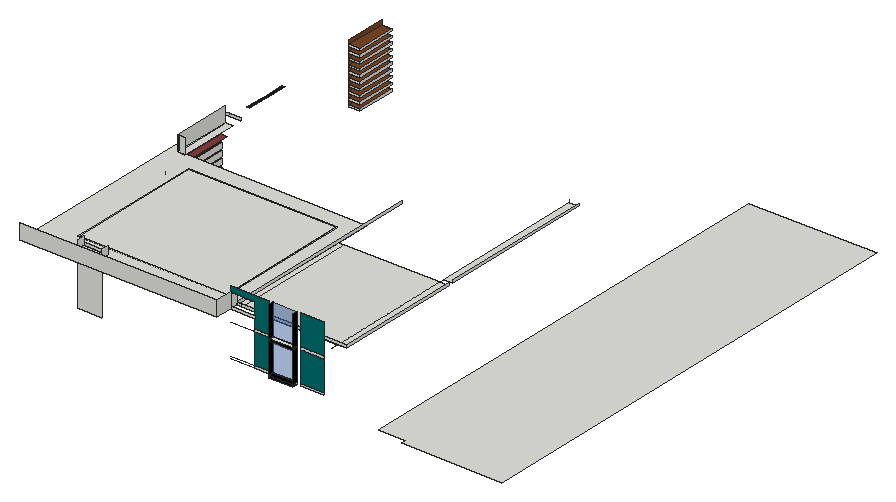
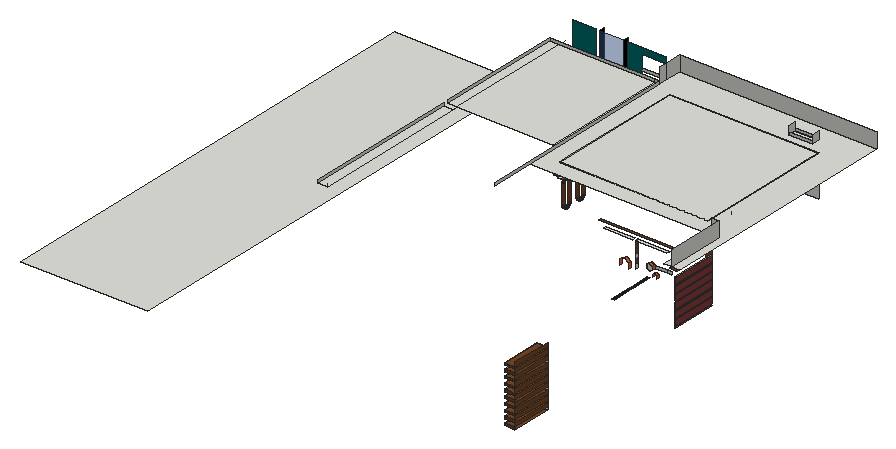
# SketchUp Ruby script. Lengths in inches.
U = 1.inch
M = Sketchup.active_model
def pt(a) = Geom::Point3d.new(a.map { |v| v * U })
def face(e, loops, mat)
  f = e.add_face(loops[0].map { |a| pt(a) })
  loops[1..].each { |l| e.add_face(l.map { |a| pt(a) }).erase! }
  f.material = f.back_material = mat if mat
  f
end
# faces: each face lists its corners as indices into pts; further lists are holes
def faces(e, pts, list, mat = nil) = list.each { |f| face(e, (f[0].is_a?(Array) ? f : [f]).map { |l| l.map { |i| pts[i] } }, mat) }
# xy, xz, yz: faces in a plane at the given z, y or x. An outline is a flat list of corners, or four numbers for a rectangle; further outlines are holes
def ring(l) = l.size == 4 ? [[l[0], l[1]], [l[2], l[1]], [l[2], l[3]], [l[0], l[3]]] : l.each_slice(2).to_a
def flat(e, list, mat, &to3) = list.each { |f| face(e, (f[0].is_a?(Array) ? f : [f]).map { |l| ring(l).map { |u, v| to3.(u, v) } }, mat) }
def xy(e, z, list, mat = nil) = flat(e, list, mat) { |x, y| [x, y, z] }
def xz(e, y, list, mat = nil) = flat(e, list, mat) { |x, z| [x, y, z] }
def yz(e, x, list, mat = nil) = flat(e, list, mat) { |y, z| [x, y, z] }
def lines(e, pts, list) = list.each { |a, b| e.add_line(pt(pts[a]), pt(pts[b])) }
# prism: a flat outline (further loops are holes) pulled along v
def prism(e, loops, v, mat = nil)
  f = face(e, loops, mat); d = Geom::Vector3d.new(v.map { |x| x * U })
  f.pushpull(f.normal.samedirection?(d) ? d.length : -d.length)
end
def box(e, o, s, mat = nil) = prism(e, [[o, [o[0] + s[0], o[1], o[2]], [o[0] + s[0], o[1] + s[1], o[2]], [o[0], o[1] + s[1], o[2]]]], [0, 0, s[2]], mat)
def at(x, y, z, deg = 0) = Geom::Transformation.translation(pt([x, y, z])) * Geom::Transformation.rotation(ORIGIN, Z_AXIS, deg.degrees)
def axes(o, x, y, z) = Geom::Transformation.new([*x, 0, *y, 0, *z, 0, *pt(o).to_a, 1])
def part(name) = M.definitions.add(name)
# library, detail: a bought-in or finely detailed component or shape, given as its bounding box
def library(name, o, s) = part(name).tap { |d| box(d.entities, o, s) }
def detail(e, o, s) = box(e.add_group.entities, o, s)
def put(e, d, t, mat = nil) = e.add_instance(d, t).tap { |i| i.material = mat if mat }
def group(e, t, mat = nil) = e.add_group.tap { |g| g.transformation = t; g.material = mat if mat }.entities
root = M.entities
M.materials.add("[0017_IndianRed]").color = [135, 60, 60]
M.materials.add("[Color A08]").color = [102, 0, 0]
M.materials.add("[Color B04]").color = [255, 101, 50]
M.materials.add("[Color C07]").color = [153, 76, 0]
M.materials.add("[Color H07]1").color = [0, 109, 109]
M.materials.add("[Color M08]").color = [30, 30, 30]
M.materials.add("[Color M09]").color = [0, 0, 0]
M.materials.add("[Translucent Glass Blue]1").color = [78, 117, 186]
M.materials["[Translucent Glass Blue]1"].alpha = 0.5
M.materials.add("[Wood Veneer 01]").color = [120, 70, 37]
xy(root,186.12,[[82.23,313.6,84.23,364.52]],"[0017_IndianRed]")
xy(root,187.92,[[77.54,552.74,89.54,598.37]],"[Wood Veneer 01]")
xy(root,188.35,[[82.23,313.6,84.23,364.52]],"[0017_IndianRed]")
xy(root,188.93,[[493.41,106.91,607.41,106.91,607.41,636.48,463.41,636.48,463.41,112.91,493.41,112.91]])
xy(root,190.33,[[77.54,552.74,89.54,598.37]],"[Wood Veneer 01]")
xy(root,194.62,[[82.23,313.6,84.23,364.52]],"[0017_IndianRed]")
xy(root,194.74,[[77.54,552.74,89.54,598.37]],"[Wood Veneer 01]")
xy(root,196.85,[[82.23,313.6,84.23,364.52]],"[0017_IndianRed]")
xy(root,197.14,[[77.54,552.74,89.54,598.37]],"[Wood Veneer 01]")
xy(root,201.55,[[77.54,552.74,89.54,598.37]],"[Wood Veneer 01]")
xy(root,202.34,[[343.08,106.91,369.95,112.91]],"[Color M09]")
xy(root,203.12,[[82.23,313.6,84.23,364.52]],"[0017_IndianRed]")
xy(root,203.95,[[77.54,552.74,89.54,598.37]],"[Wood Veneer 01]")
xy(root,204.72,[[343.08,106.91,369.95,112.91]],"[Color M09]")
xy(root,205.35,[[82.23,313.6,84.23,364.52]],"[0017_IndianRed]")
xy(root,208.36,[[77.54,552.74,89.54,598.37]],"[Wood Veneer 01]")
xy(root,210.77,[[77.54,552.74,89.54,598.37]],"[Wood Veneer 01]")
xy(root,211.62,[[82.23,313.6,84.23,364.52]],"[0017_IndianRed]")
xy(root,213.85,[[82.23,313.6,84.23,364.52]],"[0017_IndianRed]")
xy(root,215.17,[[77.54,552.74,89.54,598.37]],"[Wood Veneer 01]")
xy(root,216.61,[[139.47,302.6,175.47,305.6],[178.47,302.6,211.47,305.6]])
xy(root,217.58,[[77.54,552.74,89.54,598.37]],"[Wood Veneer 01]")
xy(root,220.12,[[82.23,313.6,84.23,364.52]],"[0017_IndianRed]")
xy(root,220.55,[[291.79,229.6,291.79,243.65,288.79,243.65,288.79,247.85,291.79,247.85,291.79,266.1,294.79,266.1,294.79,229.6]])
xy(root,220.55,[[288.79,229.6,291.79,243.65],[288.79,247.85,291.79,266.1]],"[Wood Veneer 01]")
xy(root,221.99,[[77.54,552.74,89.54,598.37]],"[Wood Veneer 01]")
xy(root,222.35,[[82.23,313.6,84.23,364.52]],"[0017_IndianRed]")
xy(root,222.61,[[133.47,302.6,217.47,305.6]],"[Wood Veneer 01]")
xy(root,224.39,[[77.54,552.74,89.54,598.37]],"[Wood Veneer 01]")
xy(root,224.91,[[291.79,170.29,294.79,183.63],[291.79,186.63,294.79,202.98]])
xy(root,226.55,[[288.79,223.6,294.79,272.1]],"[Wood Veneer 01]")
xy(root,227.91,[[291.79,167.29,294.79,205.98]],"[Color M08]")
xy(root,228.62,[[82.23,313.6,84.23,364.52]],"[0017_IndianRed]")
xy(root,228.8,[[77.54,552.74,89.54,598.37]],"[Wood Veneer 01]")
xy(root,230.85,[[82.23,313.6,84.23,364.52]],"[0017_IndianRed]")
xy(root,231.2,[[77.54,552.74,89.54,598.37]],"[Wood Veneer 01]")
xy(root,235.61,[[77.54,552.74,89.54,598.37]],"[Wood Veneer 01]")
xy(root,237.12,[[82.23,313.6,84.23,364.52]],"[0017_IndianRed]")
xy(root,238.02,[[77.54,552.74,89.54,598.37]],"[Wood Veneer 01]")
xy(root,239.34,[[343.08,106.91,369.95,112.91]],"[Color M09]")
xy(root,241.72,[[343.08,106.91,369.95,112.91]])
xy(root,242.42,[[77.54,552.74,89.54,598.37]],"[Wood Veneer 01]")
xy(root,244.62,[[80.6,313.6,82.23,364.52],[82.23,313.6,89.54,364.52]],"[0017_IndianRed]")
xy(root,244.83,[[77.54,552.74,89.54,598.37]],"[Wood Veneer 01]")
xy(root,246.61,[[[115.8,139.1875,115.8125,140.26,115.8125,279.33,268.52,279.33,268.52,139.1875],[124.47,144.14,143.78,269.32],[151.22,144.14,170.53,269.32],[177.97,144.14,197.28,269.32],[204.72,144.14,224.03,269.32],[231.47,144.14,250.78,269.32]]],"[Color A08]")
xy(root,249.24,[[77.54,552.74,89.54,598.37]],"[Wood Veneer 01]")
xy(root,249.61,[[124.47,144.14,143.78,269.32],[151.22,144.14,170.53,269.32],[177.97,144.14,197.28,269.32],[204.72,144.14,224.03,269.32],[231.47,144.14,250.78,269.32]])
xy(root,249.61,[[[107.85,131.3,107.92,140.3,107.92,287.22,276.41,287.22,276.41,131.3],[115.8,139.1875,268.52,139.1875,268.52,279.33,115.8125,279.33,115.8125,140.26]]],"[Color A08]")
xy(root,251.64,[[77.54,552.74,89.54,598.37]],"[Wood Veneer 01]")
xy(root,252.61,[[[72.04,94.04,72.04,372.52,80.6,372.52,80.6,305.6,294.79,305.6,294.79,94.04],[107.85,131.3,276.41,131.3,276.41,287.22,107.92,287.22,107.92,140.3],[121.875,112.91,149.09,121.91]],[121.875,112.91,149.09,121.91],[294.79,121.91,300.66,266.1],[300.66,121.91,300.79,266.1],[300.79,121.91,409.01,266.1],
  [409.01,121.91,419.79,266.1],[107.85,131.3,276.41,131.3,276.41,287.22,107.92,287.22,107.92,140.3],[409.01,272.1,419.79,449.91],[80.6,305.6,82.23,372.52],[82.23,305.6,89.54,372.52]])
xy(root,254.5,[[81.04,403.54,84.04,425.54],[81.04,428.54,84.04,453.54]],"[Color M08]")
xz(root,94.04,[[72.04,252.61,294.79,269.74]])
xz(root,106.91,[[343.08,202.34,369.95,204.72],[343.08,239.34,369.95,241.72]],"[Color M09]")
xz(root,112.91,[[121.875,192.65,149.09,252.61],[322.48,202.34,338.5625,204.72],[343.08,202.34,369.95,204.72],[374.46,202.34,400.27,204.72],[322.48,239.34,338.5625,241.72],
  [343.08,239.34,369.95,241.72],[374.46,239.34,400.27,241.72],[121.875,252.61,149.09,255.61],[294.79,252.61,322.48,255.61]])
xz(root,112.91,[[322.48,204.72,338.5625,239.34],[374.46,204.72,400.27,239.34],[322.48,241.72,338.5625,241.72,338.5625,276.34,294.79,276.34,294.79,269.74,322.48,269.74],[374.46,241.72,400.27,276.34]],"[Color H07]1")
xz(root,112.91,[[343.08,204.72,369.95,239.34],[343.08,241.72,369.95,276.34]],"[Translucent Glass Blue]1")
xz(root,121.91,[[121.875,252.61,149.09,255.61],[294.79,252.61,300.79,255.61],[300.79,252.61,419.79,255.61]])
xz(root,131.3,[[107.85,249.61,276.41,252.61]])
xz(root,139.1875,[[115.8,246.61,268.52,249.61]],"[Color A08]")
xz(root,144.14,[[124.47,246.61,143.78,249.61],[151.22,246.61,170.53,249.61],[177.97,246.61,197.28,249.61],[204.72,246.61,224.03,249.61],[231.47,246.61,250.78,249.61]],"[Color A08]")
xz(root,231.95,[[291.79,189.93,294.79,213.28]],"[Wood Veneer 01]")
xz(root,240.95,[[291.79,189.93,294.79,213.28]],"[Wood Veneer 01]")
xz(root,251.89,[[291.79,190.8,294.79,213.15]],"[Wood Veneer 01]")
xz(root,260.89,[[291.79,190.8,294.79,213.15]],"[Wood Veneer 01]")
xz(root,269.32,[[124.47,246.61,143.78,249.61],[151.22,246.61,170.53,249.61],[177.97,246.61,197.28,249.61],[204.72,246.61,224.03,249.61],[231.47,246.61,250.78,249.61]],"[Color A08]")
xz(root,279.33,[[115.8125,246.61,268.52,249.61]],"[Color C07]")
xz(root,287.22,[[107.92,249.61,276.41,252.61]])
xz(root,302.6,[[159.61,191.2,162.97,193.13,162.97,197.01,159.61,198.95,156.25,197.01,156.25,193.13]],"[Color B04]")
xz(root,305.6,[[159.61,191.2,156.25,193.13,156.25,197.01,159.61,198.95,162.97,197.01,162.97,193.13],[80.6,252.61,82.23,269.74],[82.23,252.61,89.54,269.74]])
xz(root,313.6,[[82.23,188.35,84.23,192.65],[82.23,192.65,84.23,194.62],[82.23,196.85,84.23,203.12],[82.23,205.35,84.23,211.62],[82.23,213.85,84.23,220.12],
  [82.23,222.35,84.23,228.62],[82.23,230.85,84.23,237.12]])
xz(root,313.6,[[84.23,192.65,84.23,194.62,82.23,194.62,82.23,196.85,84.23,196.85,84.23,203.12,82.23,203.12,82.23,205.35,84.23,205.35,84.23,211.62,82.23,211.62,82.23,213.85,84.23,213.85,84.23,220.12,82.23,220.12,82.23,222.35,84.23,222.35,84.23,228.62,82.23,228.62,82.23,230.85,84.23,230.85,84.23,237.12,82.23,237.12,82.23,244.62,89.54,244.62,89.54,192.65]],"[0017_IndianRed]")
xz(root,364.52,[[82.23,188.35,84.23,194.62],[82.23,196.85,84.23,203.12],[82.23,205.35,84.23,211.62],[82.23,213.85,84.23,220.12],[82.23,222.35,84.23,228.62],
  [82.23,230.85,84.23,237.12]])
xz(root,383.99,[[72.04,252.61,76.23,255.61],[76.23,252.61,89.54,255.61]])
xz(root,552.74,[[77.54,187.92,89.54,190.33],[77.54,194.74,89.54,197.14],[77.54,201.55,89.54,203.95],[77.54,208.36,89.54,210.77],[77.54,215.17,89.54,217.58],
  [77.54,221.99,89.54,224.39],[77.54,228.8,89.54,231.2],[77.54,235.61,89.54,238.02],[77.54,242.42,89.54,244.83],[77.54,249.24,89.54,251.64]])
xz(root,598.37,[[77.54,187.92,89.54,190.33],[77.54,194.74,89.54,197.14],[77.54,201.55,89.54,203.95],[77.54,208.36,89.54,210.77],[77.54,215.17,89.54,217.58],
  [77.54,221.99,89.54,224.39],[77.54,228.8,89.54,231.2],[77.54,235.61,89.54,238.02],[77.54,242.42,89.54,244.83],[77.54,249.24,89.54,251.64]],"[Wood Veneer 01]")
yz(root,77.54,[[552.74,190.33,598.37,194.74],[552.74,197.14,598.37,201.55],[552.74,203.95,598.37,208.36],[552.74,210.77,598.37,215.17],[552.74,217.58,598.37,221.99],
  [552.74,224.39,598.37,228.8],[552.74,231.2,598.37,235.61],[552.74,238.02,598.37,242.42],[552.74,244.83,598.37,249.24],[552.74,251.64,598.37,256.05]],"[Wood Veneer 01]")
yz(root,80.6,[[305.6,252.61,372.52,269.74]])
yz(root,82.23,[[313.6,188.35,364.52,194.62],[313.6,196.85,364.52,203.12],[313.6,205.35,364.52,211.62],[313.6,213.85,364.52,220.12],[313.6,222.35,364.52,228.62],
  [313.6,230.85,364.52,237.12]],"[0017_IndianRed]")
yz(root,84.23,[[313.6,188.35,364.52,194.62],[313.6,196.85,364.52,203.12],[313.6,205.35,364.52,211.62],[313.6,213.85,364.52,220.12],[313.6,222.35,364.52,228.62],
  [313.6,230.85,364.52,237.12]])
yz(root,89.54,[[552.74,187.92,598.37,190.33],[552.74,194.74,598.37,197.14],[552.74,201.55,598.37,203.95],[552.74,208.36,598.37,210.77],[552.74,215.17,598.37,217.58],
  [552.74,221.99,598.37,224.39],[552.74,228.8,598.37,231.2],[552.74,235.61,598.37,238.02],[552.74,242.42,598.37,244.83],[552.74,249.24,598.37,251.64]])
yz(root,107.92,[[140.3,249.61,287.22,252.61]])
yz(root,115.8125,[[140.26,246.61,279.33,249.61]],"[Color A08]")
yz(root,121.875,[[112.91,252.61,121.91,261.93]])
yz(root,124.47,[[144.14,246.61,269.32,249.61]],"[Color A08]")
yz(root,143.78,[[144.14,246.61,269.32,249.61]],"[Color A08]")
yz(root,149.09,[[112.91,252.61,121.91,261.93]])
yz(root,151.22,[[144.14,246.61,269.32,249.61]],"[Color A08]")
yz(root,151.34,[[302.6,185.9375,305.6,188.875]],"[Color B04]")
yz(root,156.25,[[302.6,193.13,305.6,197.01]],"[Color B04]")
yz(root,156.43,[[302.6,185.9375,305.6,188.875]],"[Color B04]")
yz(root,162.97,[[302.6,193.13,305.6,197.01]],"[Color B04]")
yz(root,170.53,[[144.14,246.61,269.32,249.61]],"[Color A08]")
yz(root,175.47,[[302.6,187.88,305.6,192.82],[302.6,197.75,305.6,202.69]])
yz(root,175.47,[[302.6,192.82,305.6,197.75],[302.6,202.69,305.6,216.61]],"[Wood Veneer 01]")
yz(root,177.97,[[144.14,246.61,269.32,249.61]],"[Color A08]")
yz(root,182.77,[[302.6,185.11,305.6,191.23]],"[Color B04]")
yz(root,193.38,[[302.6,185.11,305.6,191.23]],"[Color B04]")
yz(root,197.28,[[144.14,246.61,269.32,249.61]],"[Color A08]")
yz(root,204.72,[[144.14,246.61,269.32,249.61]],"[Color A08]")
yz(root,224.03,[[144.14,246.61,269.32,249.61]],"[Color A08]")
yz(root,231.47,[[144.14,246.61,269.32,249.61]],"[Color A08]")
yz(root,250.78,[[144.14,246.61,269.32,249.61]],"[Color A08]")
yz(root,268.52,[[139.1875,246.61,279.33,249.61]],"[Color A08]")
yz(root,276.41,[[131.3,249.61,266.1,252.61],[266.1,249.61,287.22,252.61]])
yz(root,294.79,[[94.04,252.61,112.91,269.74],[112.91,252.61,121.91,269.74],[121.91,252.61,355.8,255.61]])
yz(root,343.08,[[106.91,202.34,112.91,204.72],[106.91,239.34,112.91,241.72]])
yz(root,343.08,[[106.91,204.72,112.91,239.34],[106.91,241.72,112.91,276.34]],"[Color M09]")
yz(root,369.95,[[106.91,204.72,112.91,239.34],[106.91,241.72,112.91,276.34]],"[Color M09]")
yz(root,419.79,[[121.91,252.61,266.1,255.61],[272.1,252.61,449.91,255.61]])
p = [[291.79,236.45,186.16],[291.79,235.4,186.28],[294.79,235.4,186.28],[294.79,236.45,186.16],[291.79,237.5,186.28],[294.79,237.5,186.28],
  [291.79,234.4,186.65],[294.79,234.4,186.65],[291.79,238.5,186.65],[294.79,238.5,186.65],[291.79,256.39,186.3],[291.79,255.23,186.45],
  [294.79,255.23,186.45],[294.79,256.39,186.3],[291.79,257.55,186.45],[294.79,257.55,186.45],[291.79,254.14,186.9],[294.79,254.14,186.9],
  [291.79,258.64,186.9],[294.79,258.64,186.9],[291.79,233.52,187.23],[294.79,233.52,187.23],[291.79,239.39,187.23],[294.79,239.39,187.23],
  [291.79,253.21,187.61],[294.79,253.21,187.61],[291.79,259.57,187.61],[294.79,259.57,187.61],[291.79,232.79,188],[294.79,232.79,188],
  [291.79,240.11,188],[294.79,240.11,188],[291.79,252.49,188.55],[294.79,252.49,188.55],[291.79,260.29,188.55],[294.79,260.29,188.55],
  [291.79,232.26,188.91],[294.79,232.26,188.91],[291.79,240.65,188.91],[294.79,240.65,188.91],[291.79,252.04,189.63],[294.79,252.04,189.63],
  [291.79,260.74,189.63],[294.79,260.74,189.63],[291.79,231.95,189.93],[294.79,231.95,189.93],[291.79,240.95,189.93],[294.79,240.95,189.93],
  [153.89,305.6,190.34],[151.34,305.6,188.875],[151.34,302.6,188.875],[153.89,302.6,190.34],[156.43,305.6,188.875],[156.43,302.6,188.875],
  [291.79,251.89,190.8],[294.79,251.89,190.8],[291.79,260.89,190.8],[294.79,260.89,190.8],[156.25,305.6,193.13],[159.61,305.6,191.2],
  [159.61,302.6,191.2],[156.25,302.6,193.13],[162.97,305.6,193.13],[162.97,302.6,193.13],[188.08,305.6,194.3],[182.77,305.6,191.23],
  [182.77,302.6,191.23],[188.08,302.6,194.3],[193.38,305.6,191.23],[193.38,302.6,191.23],[159.61,305.6,198.95],[156.25,305.6,197.01],
  [156.25,302.6,197.01],[159.61,302.6,198.95],[162.97,305.6,197.01],[162.97,302.6,197.01],[291.79,251.89,213.15],[291.79,252.25,214.11],
  [294.79,252.25,214.11],[294.79,251.89,213.15],[291.79,260.53,214.11],[291.79,260.89,213.15],[294.79,260.89,213.15],[294.79,260.53,214.11],
  [291.79,231.95,213.28],[291.79,232.33,214.21],[294.79,232.33,214.21],[294.79,231.95,213.28],[291.79,240.57,214.21],[291.79,240.95,213.28],
  [294.79,240.95,213.28],[294.79,240.57,214.21],[291.79,252.8,214.97],[294.79,252.8,214.97],[291.79,259.98,214.97],[294.79,259.98,214.97],
  [291.79,232.9,215.04],[294.79,232.9,215.04],[291.79,240,215.04],[294.79,240,215.04],[291.79,233.64,215.72],[294.79,233.64,215.72],
  [291.79,239.27,215.72],[294.79,239.27,215.72],[291.79,253.54,215.68],[294.79,253.54,215.68],[291.79,259.24,215.68],[294.79,259.24,215.68],
  [291.79,234.5,216.24],[294.79,234.5,216.24],[291.79,238.4,216.24],[294.79,238.4,216.24],[291.79,254.41,216.22],[294.79,254.41,216.22],
  [291.79,258.375,216.22],[294.79,258.375,216.22],[291.79,235.45,216.55],[294.79,235.45,216.55],[291.79,237.45,216.55],[294.79,237.45,216.55],
  [291.79,255.375,216.55],[294.79,255.375,216.55],[291.79,257.41,216.55],[294.79,257.41,216.55],[291.79,256.39,216.66],[294.79,256.39,216.66],
  [291.79,236.45,216.66],[294.79,236.45,216.66],[115.8,139.1875,249.61],[115.8125,140.26,249.61],[115.8125,140.26,246.61],[115.8,139.1875,246.61],
  [107.85,131.3,252.61],[107.92,140.3,252.61],[107.92,140.3,249.61],[107.85,131.3,249.61],[409.01,112.91,252.61],[409.01,121.91,252.61],
  [409.01,266.1,252.61],[409.01,272.1,252.61],[409.01,449.91,252.61],[409.01,449.91,255.61],[98.54,266.1,252.61],[98.54,266.1,255.61],
  [294.79,112.91,239.34],[322.48,112.91,239.34],[294.79,112.91,202.34],[322.48,112.91,202.34],[322.48,112.91,204.72],[294.79,112.91,204.72]]
faces(root,p,[[0,1,2,3],[4,0,3,5],[1,6,7,2],[8,4,5,9],[10,11,12,13],[14,10,13,15],[11,16,17,12],[18,14,15,19],
  [6,20,21,7],[22,8,9,23],[16,24,25,17],[26,18,19,27],[20,28,29,21],[30,22,23,31],[24,32,33,25],[34,26,27,35],
  [28,36,37,29],[38,30,31,39],[32,40,41,33],[42,34,35,43],[36,44,45,37],[46,38,39,47],[40,54,55,41],[56,42,43,57],
  [76,77,78,79],[80,81,82,83],[84,85,86,87],[88,89,90,91],[77,92,93,78],[94,80,83,95],[85,96,97,86],[98,88,91,99],
  [96,100,101,97],[102,98,99,103],[92,104,105,93],[106,94,95,107],[100,108,109,101],[110,102,103,111],[104,112,113,105],[114,106,107,115],
  [108,116,117,109],[118,110,111,119],[112,120,121,113],[122,114,115,123],[120,124,125,121],[124,122,123,125],[116,126,127,117],[126,118,119,127]],"[Wood Veneer 01]")
faces(root,p,[[48,49,50,51],[52,48,51,53],[58,59,60,61],[59,62,63,60],[64,65,66,67],[68,64,67,69],[70,71,72,73],[74,70,73,75]],"[Color B04]")
faces(root,p,[[128,129,130,131]],"[Color A08]")
faces(root,p,[[132,133,134,135]])
lines(root,p,[[136,137],[138,139],[140,141],[142,143],[144,145],[146,147],[148,149]])
